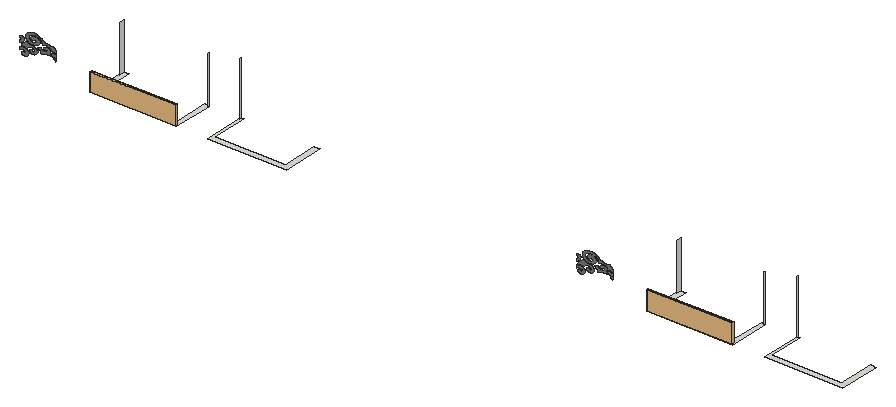
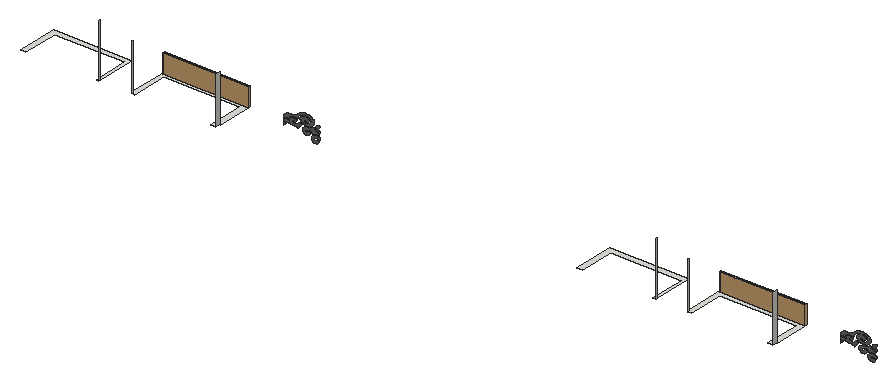
# SketchUp Ruby script. Lengths in inches.
U = 1.inch
M = Sketchup.active_model
def pt(a) = Geom::Point3d.new(a.map { |v| v * U })
def face(e, loops, mat)
  f = e.add_face(loops[0].map { |a| pt(a) })
  loops[1..].each { |l| e.add_face(l.map { |a| pt(a) }).erase! }
  f.material = f.back_material = mat if mat
  f
end
# faces: each face lists its corners as indices into pts; further lists are holes
def faces(e, pts, list, mat = nil) = list.each { |f| face(e, (f[0].is_a?(Array) ? f : [f]).map { |l| l.map { |i| pts[i] } }, mat) }
# xy, xz, yz: faces in a plane at the given z, y or x. An outline is a flat list of corners, or four numbers for a rectangle; further outlines are holes
def ring(l) = l.size == 4 ? [[l[0], l[1]], [l[2], l[1]], [l[2], l[3]], [l[0], l[3]]] : l.each_slice(2).to_a
def flat(e, list, mat, &to3) = list.each { |f| face(e, (f[0].is_a?(Array) ? f : [f]).map { |l| ring(l).map { |u, v| to3.(u, v) } }, mat) }
def xy(e, z, list, mat = nil) = flat(e, list, mat) { |x, y| [x, y, z] }
def xz(e, y, list, mat = nil) = flat(e, list, mat) { |x, z| [x, y, z] }
def yz(e, x, list, mat = nil) = flat(e, list, mat) { |y, z| [x, y, z] }
def lines(e, pts, list) = list.each { |a, b| e.add_line(pt(pts[a]), pt(pts[b])) }
# prism: a flat outline (further loops are holes) pulled along v
def prism(e, loops, v, mat = nil)
  f = face(e, loops, mat); d = Geom::Vector3d.new(v.map { |x| x * U })
  f.pushpull(f.normal.samedirection?(d) ? d.length : -d.length)
end
def box(e, o, s, mat = nil) = prism(e, [[o, [o[0] + s[0], o[1], o[2]], [o[0] + s[0], o[1] + s[1], o[2]], [o[0], o[1] + s[1], o[2]]]], [0, 0, s[2]], mat)
def at(x, y, z, deg = 0) = Geom::Transformation.translation(pt([x, y, z])) * Geom::Transformation.rotation(ORIGIN, Z_AXIS, deg.degrees)
def axes(o, x, y, z) = Geom::Transformation.new([*x, 0, *y, 0, *z, 0, *pt(o).to_a, 1])
def part(name) = M.definitions.add(name)
# library, detail: a bought-in or finely detailed component or shape, given as its bounding box
def library(name, o, s) = part(name).tap { |d| box(d.entities, o, s) }
def detail(e, o, s) = box(e.add_group.entities, o, s)
def put(e, d, t, mat = nil) = e.add_instance(d, t).tap { |i| i.material = mat if mat }
def group(e, t, mat = nil) = e.add_group.tap { |g| g.transformation = t; g.material = mat if mat }.entities
root = M.entities
M.materials.add("[0043_SaddleBrown]4").color = [124, 123, 122]
c1 = library("Glass Railing",[0,0,0],[139.5,4.76,42])
xy(root,541.1875,[[550.01,558.125,744.19,558.125,744.19,647.91,742.44,647.91,742.44,651.03,734.59,651.03,734.59,570.83,563.08,570.83,563.08,651.03,551.76,651.03,551.76,640.11,550.01,640.11],[814.68,558.125,991.94,558.125,991.94,651.03,978.86,651.03,978.86,570.83,820.97,570.83,820.97,651.03,814.68,651.03],[1800.63,558.125,1994.82,558.125,1994.82,647.91,1993.07,647.91,1993.07,651.03,1985.21,651.03,1985.21,570.83,1813.71,570.83,1813.71,651.03,1802.38,651.03,1802.38,640.11,1800.63,640.11],[2065.31,558.125,2242.56,558.125,2242.56,651.03,2229.49,651.03,2229.49,570.83,2071.59,570.83,2071.59,651.03,2065.31,651.03]])
xz(root,589.17,[[378.54,541.67,377.25,541.71,376.01,541.9,374.84,542.23,373.8,542.69,372.92,543.27,372.23,543.93,371.75,544.67,371.51,545.44,371.42,545.74,371.43,546.04,371.53,546.34,371.72,546.62,372,546.875,372.35,547.09,372.77,547.26,373.23,547.37,373.71,547.43,374.21,547.43,374.69,547.37,375.15,547.25,375.42,547.03,375.71,546.83,376.02,546.64,376.34,546.45,376.69,546.29,377.05,546.13,377.43,545.99,377.82,545.87,378.23,545.76,378.64,545.66,379.0625,545.58,379.49,545.52,380.06,545.82,380.55,546.16,380.98,546.53,381.33,546.93,381.6,547.36,381.78,547.8,381.88,548.25,381.88,548.71,381.79,549.16,381.61,549.6,381.35,550.03,381,550.43,380.27,551.04,379.38,551.56,378.37,551.98,377.25,552.29,376.0625,552.48,374.84,552.55,373.62,552.48,372.43,552.29,371.3125,551.98,370.3,551.56,369.41,551.04,368.68,550.43,368.68,554.9,369.56,555.28,370.49,555.61,371.47,555.89,372.49,556.1,373.54,556.26,374.6,556.35,375.68,556.37,376.75,556.33,377.82,556.23,378.86,556.07,379.87,555.84,380.84,555.55,382.54,554.88,384.04,554.04,385.3,553.07,386.29,551.99,386.99,550.82,387.37,549.61,387.43,548.36,387.17,547.13,386.59,545.94,385.7,544.83,384.54,543.8125,383.125,542.92,382.15,542.41,381.03,542.02,379.81,541.77],[1629.16,541.67,1627.88,541.71,1626.63,541.9,1625.47,542.23,1624.42,542.69,1623.54,543.27,1622.85,543.93,1622.375,544.67,1622.14,545.44,1622.05,545.74,1622.05,546.04,1622.15,546.34,1622.35,546.62,1622.625,546.875,1622.98,547.09,1623.39,547.26,1623.85,547.37,1624.34,547.43,1624.83,547.43,1625.32,547.37,1625.78,547.25,1626.04,547.03,1626.33,546.83,1626.64,546.64,1626.97,546.45,1627.32,546.29,1627.68,546.13,1628.06,545.99,1628.45,545.87,1628.85,545.76,1629.26,545.66,1629.6875,545.58,1630.12,545.52,1630.68,545.82,1631.18,546.16,1631.61,546.53,1631.96,546.93,1632.23,547.36,1632.41,547.8,1632.5,548.25,1632.5,548.71,1632.41,549.16,1632.24,549.6,1631.97,550.03,1631.62,550.43,1630.89,551.04,1630.01,551.56,1628.99,551.98,1627.875,552.29,1626.6875,552.48,1625.46,552.55,1624.24,552.48,1623.05,552.29,1621.9375,551.98,1620.92,551.56,1620.04,551.04,1619.31,550.43,1619.31,554.9,1620.18,555.28,1621.11,555.61,1622.09,555.89,1623.11,556.1,1624.16,556.26,1625.23,556.35,1626.3,556.37,1627.38,556.33,1628.44,556.23,1629.49,556.07,1630.5,555.84,1631.47,555.55,1633.16,554.88,1634.66,554.04,1635.92,553.07,1636.91,551.99,1637.61,550.82,1637.99,549.61,1638.06,548.36,1637.79,547.13,1637.21,545.94,1636.33,544.83,1635.16,543.8125,1633.75,542.92,1632.77,542.41,1631.65,542.02,1630.43,541.77],[398.55,551.33,396.95,551.39,395.4,551.65,393.97,552.1,392.73,552.73,391.73,553.5,391.02,554.38,390.62,555.34,390.5625,556.33,390.625,556.63,390.74,556.93,390.9,557.23,391.11,557.51,391.37,557.77,391.67,558.02,392,558.25,392.38,558.46,392.79,558.64,393.23,558.79,393.69,558.92,394.16,559.01,394.25,558.58,394.37,558.15,394.53,557.72,394.74,557.3,394.98,556.89,395.26,556.49,395.58,556.1,395.93,555.72,396.33,555.35,396.75,555,397.21,554.67,397.7,554.35,398.63,554.64,399.48,555.01,400.23,555.46,400.86,555.97,401.35,556.54,401.6875,557.15,401.875,557.78,401.9,558.42,401.76,559.06,401.47,559.68,401.02,560.26,400.4375,560.79,399.6,561.59,398.53,562.28,397.28,562.84,395.875,563.25,394.37,563.49,392.82,563.5625,391.28,563.45,389.8,563.17,388.43,562.72,387.21,562.13,386.2,561.41,385.42,560.59,385.2,560.37,385,560.14,384.81,559.91,384.63,559.68,384.46,559.45,384.31,559.21,384.17,558.97,384.04,558.72,383.92,558.47,383.82,558.23,383.73,557.97,383.66,557.72,382.97,558.29,382.16,558.79,381.27,559.24,380.29,559.61,379.24,559.9,378.14,560.11,377.01,560.23,375.86,560.27,374.72,560.22,373.59,560.08,372.5,559.86,371.46,559.56,371.67,559.82,371.87,560.09,372.03,560.37,372.17,560.65,372.29,560.94,372.37,561.23,372.43,561.53,372.46,561.82,372.47,562.12,372.44,562.41,372.39,562.71,372.3125,563,373.45,563.53,374.55,564.1,375.61,564.7,376.61,565.33,377.56,565.99,378.47,566.67,379.3125,567.39,380.11,568.12,380.84,568.88,381.51,569.66,382.12,570.46,382.67,571.27,383.28,570.61,383.99,569.98,384.8125,569.4,385.72,568.88,386.71,568.41,387.77,568.01,388.89,567.68,390.0625,567.42,391.27,567.24,392.51,567.13,393.75,567.1,394.99,567.14,397.41,566.8,399.7,566.2,401.77,565.37,403.58,564.32,405.07,563.1,406.1875,561.74,406.9,560.28,407.1875,558.77,407.04,557.24,406.46,555.76,405.48,554.36,404.11,553.09,402.98,552.39,401.64,551.85,400.14,551.49],[1649.18,551.33,1647.57,551.39,1646.02,551.65,1644.59,552.1,1643.35,552.73,1642.35,553.5,1641.64,554.38,1641.25,555.34,1641.1875,556.33,1641.25,556.63,1641.36,556.93,1641.52,557.23,1641.73,557.51,1641.99,557.77,1642.29,558.02,1642.63,558.25,1643.01,558.46,1643.41,558.64,1643.85,558.79,1644.31,558.92,1644.79,559.01,1644.87,558.58,1644.99,558.15,1645.16,557.72,1645.36,557.3,1645.6,556.89,1645.89,556.49,1646.2,556.1,1646.56,555.72,1646.95,555.35,1647.375,555,1647.83,554.67,1648.32,554.35,1649.26,554.64,1650.11,555.01,1650.86,555.46,1651.48,555.97,1651.97,556.54,1652.3125,557.15,1652.5,557.78,1652.52,558.42,1652.39,559.06,1652.09,559.68,1651.65,560.26,1651.0625,560.79,1650.22,561.59,1649.16,562.28,1647.9,562.84,1646.5,563.25,1645,563.49,1643.45,563.5625,1641.91,563.45,1640.43,563.17,1639.05,562.72,1637.84,562.13,1636.82,561.41,1636.04,560.59,1635.83,560.37,1635.62,560.14,1635.43,559.91,1635.25,559.68,1635.09,559.45,1634.93,559.21,1634.79,558.97,1634.66,558.72,1634.55,558.47,1634.45,558.23,1634.36,557.97,1634.28,557.72,1633.59,558.29,1632.79,558.79,1631.89,559.24,1630.91,559.61,1629.87,559.9,1628.77,560.11,1627.64,560.23,1626.49,560.27,1625.34,560.22,1624.21,560.08,1623.12,559.86,1622.08,559.56,1622.3,559.82,1622.49,560.09,1622.66,560.37,1622.8,560.65,1622.91,560.94,1623,561.23,1623.06,561.53,1623.09,561.82,1623.09,562.12,1623.07,562.41,1623.02,562.71,1622.9375,563,1624.08,563.53,1625.18,564.1,1626.23,564.7,1627.24,565.33,1628.19,565.99,1629.09,566.67,1629.9375,567.39,1630.73,568.12,1631.46,568.88,1632.14,569.66,1632.75,570.46,1633.29,571.27,1633.9,570.61,1634.62,569.98,1635.4375,569.4,1636.34,568.88,1637.33,568.41,1638.4,568.01,1639.52,567.68,1640.6875,567.42,1641.9,567.24,1643.13,567.13,1644.375,567.1,1645.62,567.14,1648.04,566.8,1650.32,566.2,1652.4,565.37,1654.21,564.32,1655.69,563.1,1656.8125,561.74,1657.52,560.28,1657.8125,558.77,1657.67,557.24,1657.09,555.76,1656.1,554.36,1654.73,553.09,1653.6,552.39,1652.26,551.85,1650.76,551.49],[449.07,553.96,448.79,554.34,448.5,554.71,448.2,555.08,447.88,555.4375,447.55,555.8,447.21,556.15,446.86,556.5,446.5,556.85,446.12,557.19,445.73,557.53,445.34,557.86,444.93,558.1875,445.2,558.35,445.5,558.5,445.81,558.64,446.13,558.76,446.47,558.86,446.83,558.95,447.1875,559.03,447.56,559.09,447.93,559.13,448.3125,559.15,448.69,559.16,449.07,559.15],
  [1699.7,553.96,1699.42,554.34,1699.125,554.71,1698.82,555.08,1698.51,555.4375,1698.18,555.8,1697.84,556.15,1697.12,556.85,1696.75,557.19,1696.36,557.53,1695.96,557.86,1695.55,558.1875,1695.83,558.35,1696.12,558.5,1696.43,558.64,1696.76,558.76,1697.1,558.86,1697.45,558.95,1697.8125,559.03,1698.18,559.09,1698.56,559.13,1698.9375,559.15,1699.32,559.16,1699.7,559.15],[416.03,558.48,415.91,559.39,415.68,560.29,415.34,561.18,414.9,562.05,414.35,562.9,413.69,563.72,412.94,564.51,412.1,565.26,411.16,565.97,410.15,566.63,409.05,567.25,407.88,567.8125,408.5,567.99,409.11,568.17,409.72,568.36,410.32,568.55,411.5,568.97,412.08,569.18,412.65,569.41,413.21,569.64,413.77,569.88,414.32,570.125,414.86,570.38,414.96,569.18,415.49,568.03,416.41,566.98,417.68,566.07,419.25,565.36,421.02,564.87,422.93,564.625,424.88,564.65,426.77,564.93,428.52,565.45,430.05,566.2,431.27,567.13,431.3,567.42,431.32,567.71,431.33,568,431.32,568.29,431.3,568.58,431.26,568.87,431.21,569.16,431.15,569.45,431.07,569.73,430.98,570.02,430.87,570.3,430.75,570.58,430.16,570.74,429.53,570.84,428.88,570.875,428.24,570.85,427.61,570.76,427.01,570.61,426.45,570.4,425.96,570.14,425.54,569.84,425.2,569.5,424.96,569.13,424.82,568.74,424.41,568.85,424.02,568.97,423.64,569.11,423.27,569.26,422.93,569.43,422.59,569.61,422.28,569.8,421.99,570,421.72,570.22,421.47,570.44,421.25,570.68,421.05,570.92,421.64,571.87,422.53,572.73,423.6875,573.46,425.0625,574.03,426.6,574.42,428.24,574.6,429.9,574.58,431.51,574.35,433.02,573.91,434.35,573.3,435.45,572.54,436.27,571.65,435.71,570.85,435.26,570.02,434.9375,569.17,434.74,568.3125,434.66,567.44,434.71,566.57,434.89,565.7,435.1875,564.85,435.61,564.02,436.15,563.21,436.81,562.4375,437.57,561.7,435.69,561.8,433.81,561.83,431.92,561.79,430.04,561.68,428.18,561.51,426.34,561.27,424.52,560.96,422.73,560.59,420.98,560.15,419.28,559.66,417.63,559.1],[1666.66,558.48,1666.54,559.39,1666.31,560.29,1665.97,561.18,1665.52,562.05,1664.97,562.9,1664.32,563.72,1663.57,564.51,1662.72,565.26,1661.79,565.97,1660.77,566.63,1659.67,567.25,1658.51,567.8125,1659.125,567.99,1659.74,568.17,1660.94,568.55,1662.12,568.97,1662.7,569.18,1663.84,569.64,1664.39,569.88,1664.94,570.125,1665.48,570.38,1665.59,569.18,1666.11,568.03,1667.04,566.98,1668.31,566.07,1669.87,565.36,1671.65,564.87,1673.56,564.625,1675.5,564.65,1677.4,564.93,1679.15,565.45,1680.67,566.2,1681.89,567.13,1681.93,567.42,1681.95,567.71,1681.96,568,1681.95,568.29,1681.93,568.58,1681.89,568.87,1681.84,569.16,1681.78,569.45,1681.7,569.73,1681.6,570.02,1681.5,570.3,1681.38,570.58,1680.78,570.74,1680.16,570.84,1679.51,570.875,1678.86,570.85,1678.23,570.76,1677.63,570.61,1677.08,570.4,1676.59,570.14,1676.17,569.84,1675.83,569.5,1675.59,569.13,1675.44,568.74,1675.04,568.85,1674.64,568.97,1674.26,569.11,1673.9,569.26,1673.55,569.43,1673.22,569.61,1672.91,569.8,1672.62,570,1672.35,570.22,1672.1,570.44,1671.875,570.68,1671.67,570.92,1672.26,571.87,1673.15,572.73,1674.3125,573.46,1675.6875,574.03,1677.23,574.42,1678.86,574.6,1680.52,574.58,1682.14,574.35,1683.64,573.91,1684.98,573.3,1686.07,572.54,1686.9,571.65,1686.33,570.85,1685.89,570.02,1685.5625,569.17,1685.36,568.3125,1685.29,567.44,1685.34,566.57,1685.51,565.7,1685.8125,564.85,1686.24,564.02,1686.78,563.21,1687.43,562.4375,1688.2,561.7,1686.32,561.8,1684.43,561.83,1682.55,561.79,1680.67,561.68,1678.81,561.51,1676.96,561.27,1675.14,560.96,1673.36,560.59,1671.61,560.15,1669.91,559.66,1668.25,559.1],[444.85,561.42,443.76,561.51,442.69,561.71,441.7,562.01,440.79,562.41,440,562.89,439.35,563.4375,438.84,564.04,438.5,564.69,438.24,564.99,438.08,565.31,438.03,565.64,438.08,565.97,438.23,566.29,438.49,566.59,438.82,566.85,439.24,567.07,439.72,567.23,440.23,567.33,440.77,567.375,441.32,567.35,441.78,567.29,442.23,567.21,442.67,567.1,443.09,566.96,443.49,566.81,443.87,566.63,444.21,566.43,444.53,566.22,444.82,565.98,445.07,565.74,445.29,565.48,445.46,565.21,445.81,565.32,446.15,565.45,446.48,565.58,446.8,565.71,447.12,565.86,447.72,566.16,448.01,566.33,448.29,566.5,448.5625,566.67,448.82,566.85,449.07,567.04,449.07,562.11,448.1,561.78,447.05,561.56,445.96,561.43],[1695.48,561.42,1694.38,561.51,1693.32,561.71,1692.32,562.01,1691.42,562.41,1690.63,562.89,1689.97,563.4375,1689.46,564.04,1689.12,564.69,1688.87,564.99,1688.71,565.31,1688.65,565.64,1688.7,565.97,1688.86,566.29,1689.11,566.59,1689.45,566.85,1689.87,567.07,1690.34,567.23,1690.86,567.33,1691.4,567.375,1691.94,567.35,1692.41,567.29,1692.86,567.21,1693.3,567.1,1693.72,566.96,1694.12,566.81,1694.49,566.63,1694.84,566.43,1695.16,566.22,1695.44,565.98,1695.7,565.74,1695.91,565.48,1696.09,565.21,1696.43,565.32,1696.77,565.45,1697.43,565.71,1698.05,566.01,1698.35,566.16,1698.64,566.33,1698.92,566.5,1699.1875,566.67,1699.45,566.85,1699.7,567.04,1699.7,562.11,1698.72,561.78,1697.68,561.56,1696.59,561.43],
  [368.68,564.47,368.68,568.51,369.77,568.79,370.73,569.2,371.53,569.74,372.13,570.36,372.5,571.04,372.625,571.76,372.5,572.48,372.13,573.17,371.53,573.79,370.73,574.32,369.77,574.73,368.68,575.01,368.68,578.44,369.93,578.38,371.15,578.2,372.3125,577.92,373.39,577.52,374.36,577.03,375.19,576.46,375.875,575.8125,376.39,575.11,376.73,574.37,376.88,573.61,376.85,572.84,376.62,572.08,376.27,571.34,375.86,570.62,375.39,569.91,374.85,569.22,374.27,568.55,373.62,567.89,372.92,567.26,372.17,566.65,371.37,566.0625,370.52,565.5,369.62,564.97],[1619.31,564.47,1619.31,568.51,1620.39,568.79,1621.36,569.2,1622.15,569.74,1622.75,570.36,1623.125,571.04,1623.25,571.76,1623.125,572.48,1622.75,573.17,1622.15,573.79,1621.36,574.32,1620.39,574.73,1619.31,575.01,1619.31,578.44,1620.56,578.38,1621.78,578.2,1622.9375,577.92,1624.01,577.52,1624.98,577.03,1625.82,576.46,1626.5,575.8125,1627.02,575.11,1627.36,574.37,1627.51,573.61,1627.47,572.84,1627.24,572.08,1626.89,571.34,1626.48,570.62,1626.01,569.91,1625.48,569.22,1624.89,568.55,1624.25,567.89,1623.55,567.26,1622.8,566.65,1621.99,566.0625,1621.14,565.5,1620.25,564.97],[449.07,568.52,448.71,569.11,448.21,569.67,447.59,570.17,446.86,570.62,446.04,571,445.13,571.3125,444.17,571.54,443.16,571.68,442.13,571.73,441.1,571.69,440.09,571.57,439.12,571.36,438.67,572.72,437.86,574.02,436.69,575.22,435.22,576.27,433.47,577.15,431.5,577.84,429.37,578.31,427.13,578.55,424.87,578.55,422.64,578.32,420.5,577.85,418.53,577.17,418.47,578.89,418,580.59,417.14,582.23,415.89,583.77,414.3,585.19,412.39,586.45,410.2,587.53,407.79,588.4,405.1875,589.05,402.46,589.45,399.67,589.61,396.87,589.52,394.42,588.91,392.2,588.01,390.31,586.87,388.82,585.52,387.77,584.03,387.22,582.4375,387.18,580.81,387.64,579.21,388.61,577.6875,390.03,576.31,391.86,575.14,394.02,574.19,395.41,573.82,396.91,573.62,398.43,573.61,399.93,573.8,401.33,574.17,402.58,574.7,403.625,575.38,404.42,576.18,404.9375,577.0625,405.15,577.99,405.05,578.93,404.65,579.83,404.37,580.16,403.99,580.45,403.53,580.69,403,580.87,402.42,580.98,401.81,581.02,401.21,580.98,400.63,580.87,400.1,580.69,399.64,580.45,399.26,580.16,398.98,579.83,398.84,579.64,398.68,579.45,398.5,579.28,398.29,579.11,398.06,578.95,397.81,578.8125,397.54,578.68,397.25,578.57,396.95,578.46,396.64,578.38,396.32,578.31,395.99,578.25,395.41,578.46,394.875,578.72,394.39,579.01,393.97,579.33,393.62,579.69,393.34,580.0625,393.14,580.46,393.02,580.87,392.98,581.28,393.02,581.69,393.15,582.1,393.36,582.49,393.75,583.02,394.23,583.52,394.79,583.99,395.43,584.42,396.15,584.8,396.92,585.13,397.75,585.41,398.63,585.63,399.54,585.8,400.47,585.9,401.41,585.94,402.36,585.92,403.85,585.78,405.3,585.51,406.67,585.13,407.95,584.64,409.12,584.05,410.14,583.36,411.01,582.6,411.7,581.78,412.21,580.91,412.53,580,412.65,579.08,412.56,578.15,411.95,576.76,411.03,575.43,409.8125,574.2,408.32,573.09,406.59,572.12,404.64,571.31,402.54,570.67,400.3,570.23,397.99,569.99,395.64,569.95,393.3125,570.11,391.04,570.48,388.85,571.41,386.87,572.5,385.13,573.73,383.67,575.1,382.51,576.57,381.67,578.12,381.17,579.73,381.01,581.36,381.1875,582.99,381.71,584.59,382.57,586.14,383.74,587.6,385.55,589.2,387.77,590.58,390.34,591.72,393.18,592.57,396.21,593.12,399.36,593.34,402.52,593.23,405.6,592.8,408.52,592.05,411.19,591.01,413.54,589.71,415.5,588.1875,416.04,587.55,416.63,586.9375,417.27,586.34,417.95,585.76,418.67,585.2,419.44,584.66,420.25,584.14,421.1,583.65,421.98,583.1875,422.9,582.75,423.85,582.33,424.83,581.95,426.13,581.57,427.47,581.23,428.83,580.94,430.22,580.7,431.625,580.5,433.05,580.36,434.48,580.26,435.92,580.2,437.36,580.2,438.8,580.25,440.23,580.34,441.66,580.49,442.21,579.94,442.78,579.4,443.36,578.86,443.95,578.33,444.55,577.81,445.17,577.28,445.79,576.77,447.07,575.75,447.73,575.25,448.4,574.75,449.07,574.26],[1699.7,568.52,1699.33,569.11,1698.83,569.67,1698.21,570.17,1697.49,570.62,1696.66,571,1695.76,571.3125,1694.79,571.54,1693.79,571.68,1692.76,571.73,1691.73,571.69,1690.72,571.57,1689.74,571.36,1689.3,572.72,1688.48,574.02,1687.32,575.22,1685.84,576.27,1684.09,577.15,1682.12,577.84,1679.99,578.31,1677.76,578.55,1675.49,578.55,1673.26,578.32,1671.13,577.85,1669.15,577.17,1669.09,578.89,1668.625,580.59,1667.76,582.23,1666.52,583.77,1664.93,585.19,1663.02,586.45,1660.83,587.53,1658.41,588.4,1655.8125,589.05,1653.09,589.45,1650.3,589.61,1647.5,589.52,1645.04,588.91,1642.83,588.01,1640.94,586.87,1639.44,585.52,1638.4,584.03,1637.84,582.4375,1637.8,580.81,1638.27,579.21,1639.23,577.6875,1640.65,576.31,1642.48,575.14,1644.64,574.19,1646.04,573.82,1647.53,573.62,1649.06,573.61,1650.55,573.8,1651.95,574.17,1653.2,574.7,1654.25,575.38,1655.05,576.18,1655.5625,577.0625,1655.78,577.99,1655.68,578.93,1655.27,579.83,1655,580.16,1654.62,580.45,1654.15,580.69,1653.62,580.87,1653.04,580.98,1652.44,581.02,1651.84,580.98,1651.26,580.87,1650.72,580.69,1650.26,580.45,1649.88,580.16,1649.61,579.83,1649.47,579.64,1649.31,579.45,1649.12,579.28,1648.91,579.11,1648.68,578.95,1648.43,578.8125,1648.16,578.68,1647.88,578.57,1647.58,578.46,1647.27,578.38,1646.94,578.31,1646.61,578.25,1646.03,578.46,1645.5,578.72,1645.02,579.01,1644.6,579.33,1644.25,579.69,1643.97,580.0625,1643.77,580.46,1643.65,580.87,1643.61,581.28,1643.65,581.69,1643.78,582.1,1643.98,582.49,1644.37,583.02,1644.85,583.52,1645.42,583.99,1646.06,584.42,1646.77,584.8,1647.55,585.13,1648.38,585.41,1649.25,585.63,1650.16,585.8,1651.09,585.9,1652.04,585.94,1652.98,585.92,1654.47,585.78,1655.92,585.51,1657.3,585.13,1658.58,584.64,1659.74,584.05,1660.77,583.36,1661.63,582.6,1662.33,581.78,1662.84,580.91,1663.15,580,1663.27,579.08,1663.18,578.15,1662.58,576.76,1661.66,575.43,1660.4375,574.2,1658.94,573.09,1657.21,572.12,1655.27,571.31,1653.16,570.67,1650.93,570.23,1648.61,569.99,1646.27,569.95,1643.9375,570.11,1641.67,570.48,1639.47,571.41,1637.49,572.5,1635.76,573.73,1634.3,575.1,1633.14,576.57,1632.3,578.12,1631.79,579.73,1631.63,581.36,1631.8125,582.99,1632.34,584.59,1633.19,586.14,1634.37,587.6,1636.17,589.2,1638.39,590.58,1640.96,591.72,1643.8,592.57,1646.84,593.12,1649.98,593.34,1653.14,593.23,1656.22,592.8,1659.14,592.05,1661.82,591.01,1664.17,589.71,1666.125,588.1875,1666.67,587.55,1667.26,586.9375,1667.89,586.34,1668.57,585.76,1669.3,585.2,1670.07,584.66,1670.875,584.14,1671.72,583.65,1672.6,583.1875,1673.52,582.75,1674.47,582.33,1675.46,581.95,1676.76,581.57,1678.09,581.23,1679.46,580.94,1680.84,580.7,1682.25,580.5,1683.67,580.36,1685.1,580.26,1686.54,580.2,1687.99,580.2,1689.43,580.25,1690.86,580.34,1692.28,580.49,1692.84,579.94,1693.41,579.4,1693.99,578.86,1694.58,578.33,1695.18,577.81,1695.79,577.28,1697.05,576.26,1697.7,575.75,1698.35,575.25,1699.02,574.75,1699.7,574.26]],"[0043_SaddleBrown]4")
xz(root,651.03,[[814.68,541.1875,814.89,662.4375],[2065.31,541.1875,2065.52,662.4375]])
yz(root,551.76,[[640.11,541.1875,651.03,646.4375]])
yz(root,742.44,[[647.91,541.1875,651.03,646.4375]])
yz(root,814.68,[[648.85,541.1875,651.03,662.4375]])
yz(root,1802.38,[[640.11,541.1875,651.03,646.4375]])
yz(root,1993.07,[[647.91,541.1875,651.03,646.4375]])
yz(root,2065.31,[[648.85,541.1875,651.03,662.4375]])
p = [[431.98,589.17,546.54],[431.89,589.17,547],[1682.6,589.17,546.54],[1682.52,589.17,547]]
lines(root,p,[[0,1],[2,3]])
put(root,c1,axes([550.01,558.125,541.1875],[1.37946,0,0],[0,1,0],[0,0,1]))
put(root,c1,axes([1800.63,558.125,541.1875],[1.37946,0,0],[0,1,0],[0,0,1]))
